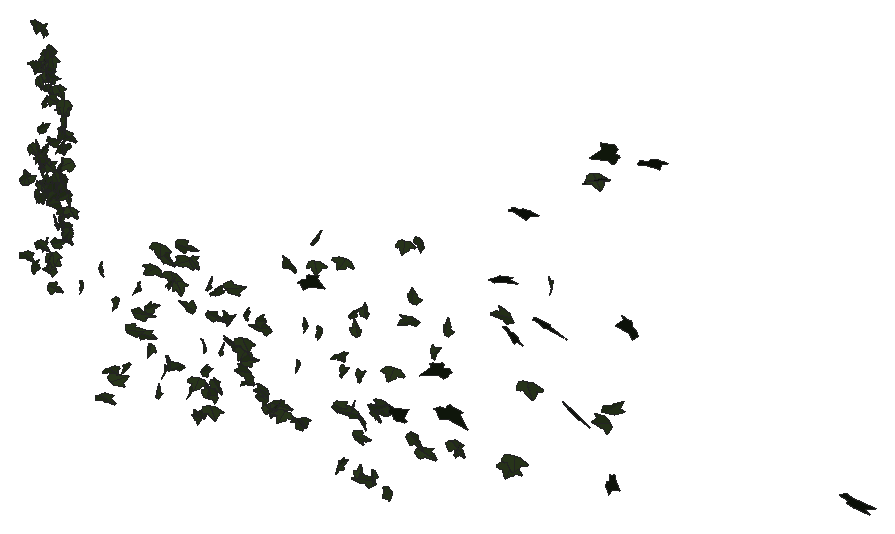
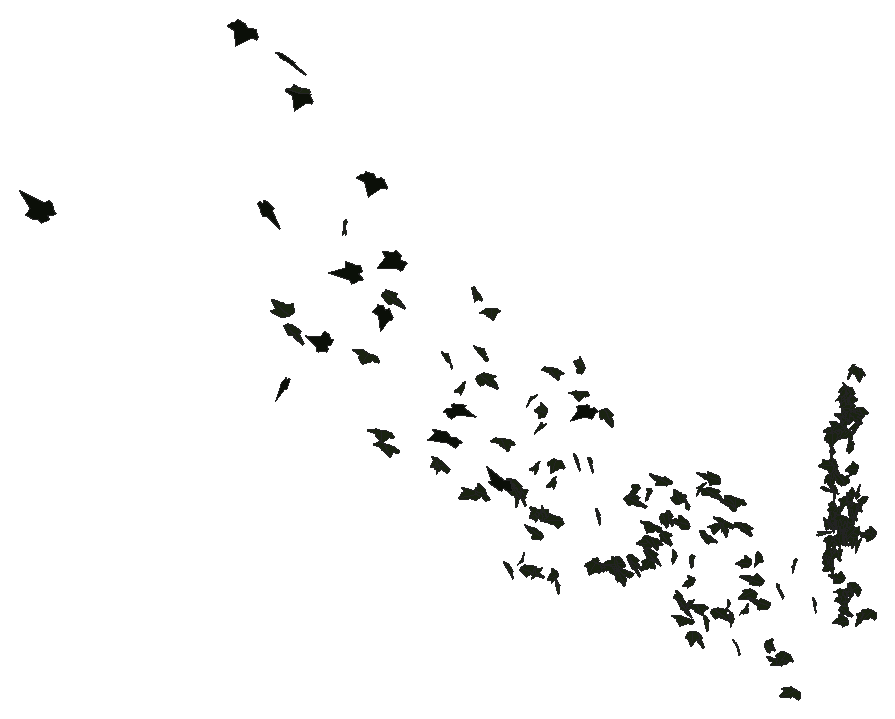
# SketchUp Ruby script. Lengths in millimetres.
U = 1.mm
M = Sketchup.active_model
def pt(a) = Geom::Point3d.new(a.map { |v| v * U })
def face(e, loops, mat)
  f = e.add_face(loops[0].map { |a| pt(a) })
  loops[1..].each { |l| e.add_face(l.map { |a| pt(a) }).erase! }
  f.material = f.back_material = mat if mat
  f
end
# faces: each face lists its corners as indices into pts; further lists are holes
def faces(e, pts, list, mat = nil) = list.each { |f| face(e, (f[0].is_a?(Array) ? f : [f]).map { |l| l.map { |i| pts[i] } }, mat) }
# xy, xz, yz: faces in a plane at the given z, y or x. An outline is a flat list of corners, or four numbers for a rectangle; further outlines are holes
def ring(l) = l.size == 4 ? [[l[0], l[1]], [l[2], l[1]], [l[2], l[3]], [l[0], l[3]]] : l.each_slice(2).to_a
def flat(e, list, mat, &to3) = list.each { |f| face(e, (f[0].is_a?(Array) ? f : [f]).map { |l| ring(l).map { |u, v| to3.(u, v) } }, mat) }
def xy(e, z, list, mat = nil) = flat(e, list, mat) { |x, y| [x, y, z] }
def xz(e, y, list, mat = nil) = flat(e, list, mat) { |x, z| [x, y, z] }
def yz(e, x, list, mat = nil) = flat(e, list, mat) { |y, z| [x, y, z] }
def lines(e, pts, list) = list.each { |a, b| e.add_line(pt(pts[a]), pt(pts[b])) }
# prism: a flat outline (further loops are holes) pulled along v
def prism(e, loops, v, mat = nil)
  f = face(e, loops, mat); d = Geom::Vector3d.new(v.map { |x| x * U })
  f.pushpull(f.normal.samedirection?(d) ? d.length : -d.length)
end
def box(e, o, s, mat = nil) = prism(e, [[o, [o[0] + s[0], o[1], o[2]], [o[0] + s[0], o[1] + s[1], o[2]], [o[0], o[1] + s[1], o[2]]]], [0, 0, s[2]], mat)
def at(x, y, z, deg = 0) = Geom::Transformation.translation(pt([x, y, z])) * Geom::Transformation.rotation(ORIGIN, Z_AXIS, deg.degrees)
def axes(o, x, y, z) = Geom::Transformation.new([*x, 0, *y, 0, *z, 0, *pt(o).to_a, 1])
def part(name) = M.definitions.add(name)
# library, detail: a bought-in or finely detailed component or shape, given as its bounding box
def library(name, o, s) = part(name).tap { |d| box(d.entities, o, s) }
def detail(e, o, s) = box(e.add_group.entities, o, s)
def put(e, d, t, mat = nil) = e.add_instance(d, t).tap { |i| i.material = mat if mat }
def group(e, t, mat = nil) = e.add_group.tap { |g| g.transformation = t; g.material = mat if mat }.entities
root = M.entities
M.materials.add("efeu1").color = [18, 25, 13]
M.materials.add("efeu2").color = [43, 57, 29]
c1 = part("ivyleaf_10")
p = [[0,12.8,-0.8],[-1.5,51.3,-10.9],[-4.9,51,-11.6],[-13.6,26.5,-7.3],[-13.2,15.9,-4.6],[-21.1,19.3,-7.2],
  [-29.5,16.3,-8.3],[-29.2,8.3,-6.2],[-19.7,-9.8,0.5],[-7.6,-13,4],[1,-12.2,5.8],[-0.4,51.1,-11.1],
  [-1.5,51.1,-10.9],[1,-12.4,5.9],[16.9,-12.4,3.5],[35.1,9.1,-5.1],[35,12.9,-6.1],[20.5,16.4,-4.9],
  [15.8,15,-3.8],[15.3,27.6,-7.1],[12.8,31.3,-7.8]]
faces(c1.entities,p,[[0,1,2,3,4,5,6,7,8,9,10],[11,12,0,13,14,15,16,17,18,19,20]],"efeu2")
c2 = part("ivyleaf_9")
p = [[39.1,54.8,31.7],[34.5,51.8,30.2],[-5.3,25.2,17.3],[-17.9,28.3,20.9],[-21.6,21.7,17],[-20.2,4.3,5.3],
  [-22.9,-0.3,2.5],[-17.1,-4,-0.6],[-2,-2.1,-1.2],[-0.7,-15.4,-10.1],[16.6,-22.3,-16.7],[21.1,-15.1,-12.5],
  [32.7,-10.7,-11],[46.1,-1.8,-6.6],[30.8,11.2,3.8]]
faces(c2.entities,p,[[0,1,2,3,4,5,6,7,8,9,10,11,12,13,14]],"efeu1")
put(root,c1,axes([1417.2,1060.7,237.2],[0.00481,0.00823,0.65497],[-0.143,0.65065,-0.00789],[-1.2384,-0.0751,0.00345]))
put(root,c1,axes([847.1,1071.3,767.4],[0.27579,-0.61594,-0.22684],[-0.01202,0.23671,-0.65255],[0.8007,0.21571,0.06834]))
put(root,c2,axes([2730.5,1072.8,870.6],[1.36099,-0.29359,0.30538],[0.54746,-0.10333,-0.77292],[0.59187,0.77069,0.0127]))
put(root,c1,axes([1434.3,1071.8,440],[0.24904,-0.04769,0.62357],[1.1423,0.18856,-0.11153],[-0.33439,0.60861,0.08342]))
put(root,c1,axes([1433.5,1072.7,105.2],[1.05934,0.28952,0.18915],[0.31871,0.08794,-0.62741],[-0.57587,0.58126,0.00071]))
put(root,c1,axes([1847.2,1066,846.2],[0.34798,-0.60012,0.45518],[-0.14943,0.45066,0.6257],[-1.42571,-0.19371,0.04552]))
put(root,c1,axes([1718.8,1076.8,188.1],[0.90095,0.37363,-0.23743],[-0.35141,-0.14928,-0.60307],[-0.76574,0.50812,-0.00259]))
put(root,c1,axes([843.6,1070.7,828.9],[0.01979,-0.64952,-0.24261],[0.13234,0.24206,-0.64081],[0.83547,-0.02296,0.10725]))
put(root,c1,axes([1582,1061.5,493.4],[-0.02885,0.10194,0.6291],[-0.48234,0.57642,-0.09951],[-1.11289,-0.25247,0.02682]))
put(root,c1,axes([832.4,1066.8,542.8],[-0.36855,0.38808,-0.44475],[-0.31395,0.36304,0.49158],[0.64808,0.39656,-0.01478]))
put(root,c1,axes([1339.1,1077,594.4],[0.92186,0.07712,-0.4767],[-0.89317,-0.08395,-0.49043],[-0.2166,0.6744,-0.00653]))
put(root,c1,axes([1194.9,1062.3,381.9],[-0.05109,-0.13598,0.63034],[0.0985,0.6284,0.13776],[-1.2233,0.05628,-0.01523]))
put(root,c2,axes([1823.8,1062.2,704.9],[0.06022,-0.12649,-0.76017],[-0.18241,0.75426,-0.12949],[1.45526,0.09978,0.01523]))
put(root,c1,axes([851.6,1074.5,982.4],[0.52934,0.52433,-0.07138],[-0.05892,-0.05268,-0.68056],[-0.64288,0.43655,0.00361]))
put(root,c1,axes([1649.9,1067.2,226.8],[0.5581,-0.38266,-0.5931],[-0.69671,0.46666,-0.48208],[1.14853,0.46902,-0.00423]))
put(root,c1,axes([1099.1,1084.1,135],[0.12569,-0.45119,0.46437],[0.08625,-0.46241,-0.45573],[1.22923,0.07858,-0.0155]))
put(root,c1,axes([1178.8,1066,283.4],[-0.45772,-0.26948,-0.52768],[0.68844,0.38427,-0.36111],[0.89313,-0.43431,0.00791]))
put(root,c1,axes([2627.1,1075.1,346.6],[1.37258,0.27698,0.03221],[0.05707,0.01177,-0.77256],[-0.52763,0.72182,0.00023]))
put(root,c1,axes([2388.3,1077,315],[0.93628,-0.01391,0.55242],[1.04983,-0.0318,-0.49203],[0.06279,0.73904,-0.01077]))
put(root,c1,axes([1559.3,1074.1,389.2],[1.13118,0.14862,0.25352],[0.45961,0.07893,-0.61243],[-0.31871,0.64133,0.01662]))
put(root,c1,axes([1452.1,1074.9,519.5],[-0.33025,-0.63394,0.08937],[0.05216,0.08516,0.65725],[-1.21733,0.17563,0.00391]))
put(root,c1,axes([744.3,1074.3,1085.4],[-0.66863,-0.33572,0.07291],[-0.0848,-0.02607,-0.64256],[0.41046,-0.55227,-0.01399]))
put(root,c1,axes([1631.8,1062.3,490.4],[0.03397,0.25278,0.58916],[-0.17207,0.58449,-0.24804],[-1.20793,-0.07615,0.0519]))
put(root,c1,axes([1057.8,1067.1,78.9],[0.73804,0.02328,-0.51446],[0.85489,0.29969,0.35215],[0.47937,-0.5703,0.16405]))
put(root,c1,axes([2047.3,1064.8,658.8],[0.1271,0.53267,-0.42449],[-0.00484,0.42672,0.53507],[1.29631,-0.05063,0.04362]))
put(root,c1,axes([777.1,1065.3,1221.3],[-0.2531,0.53421,0.39539],[-0.16532,0.3715,-0.57304],[-0.79379,-0.2477,-0.00672]))
put(root,c1,axes([1243.8,1079.5,576.9],[0.36883,-0.02855,0.63402],[1.17176,-0.15246,-0.19505],[0.2932,0.64521,-0.01804]))
put(root,c1,axes([1578,1069.6,287.9],[0.65752,-0.25995,-0.6108],[-0.89974,0.38703,-0.43212],[0.8869,0.58536,0.01446]))
put(root,c1,axes([867,1084.2,770.2],[-0.75924,0.29011,0.36104],[-0.51572,-0.6029,-0.24419],[0.23091,-0.39263,0.64174]))
put(root,c1,axes([2070.5,1080.7,99.9],[-0.04522,0.55589,-0.39749],[0.00246,-0.3977,-0.55625],[-1.30061,-0.02008,0.01277]))
put(root,c1,axes([1042.7,1070.5,111.8],[-0.69334,-0.43342,-0.3087],[0.41708,0.21872,-0.56569],[0.92285,-0.42447,0.02373]))
put(root,c1,axes([2787,1059.6,1017.5],[0.12788,-0.15203,-0.82381],[-0.14117,0.82213,-0.15777],[1.58809,0.08533,0.05231]))
put(root,c1,axes([2026.5,1061.5,432.2],[0.10352,0.0674,-0.67068],[0.2713,0.6565,0.07754],[1.25386,-0.14761,0.0386]))
put(root,c1,axes([1700.4,1072.7,218.8],[-0.00793,-0.63198,-0.20325],[-0.00251,0.20326,-0.63199],[1.26346,-0.00356,-0.00253]))
put(root,c1,axes([871.1,1081.8,609.4],[-0.33773,-0.62901,0.01414],[0.75646,-0.27537,-0.11044],[0.13021,-0.03172,0.6783]))
put(root,c1,axes([748.2,1075.3,1225.8],[-0.81266,0.06782,0.13447],[-0.17703,-0.12568,-0.65539],[-0.04921,-0.66783,0.137]))
put(root,c1,axes([757.4,1072.8,453.6],[-0.54125,-0.03239,-0.53298],[0.64951,0.02646,-0.44476],[0.0501,-0.69296,0.00793]))
put(root,c1,axes([804.2,1084.5,639.2],[-0.17556,-0.45275,0.43683],[-0.06899,-0.43699,-0.47154],[0.76443,-0.14341,0.05777]))
put(root,c1,axes([1422.6,1067.5,154.4],[0.03332,0.5523,-0.32851],[-0.01654,0.3288,0.55233],[1.22291,-0.0106,0.01642]))
put(root,c1,axes([2410.9,1063,298.1],[0.22768,-0.23907,0.6877],[-0.47086,0.6421,0.26625],[-1.3032,-0.27376,0.02394]))
put(root,c1,axes([1510.5,1070.8,560.1],[0.61861,0.02522,-0.59187],[1.09941,0.1362,0.32304],[0.24999,-0.66137,0.04396]))
put(root,c1,axes([1313.7,1074.2,643.3],[-0.05035,0.01832,-0.68042],[1.2934,-0.0376,-0.02743],[-0.07289,-0.6799,-0.01681]))
put(root,c1,axes([1255.7,1068.5,179.3],[0.17291,-0.50518,-0.45873],[-0.09673,0.45648,-0.51277],[1.2951,0.10154,0.02295]))
put(root,c1,axes([2019.2,1077.9,277.4],[-0.71041,0.48049,-0.3051],[0.32241,-0.25453,-0.60811],[-1.03416,-0.40942,0.02]))
put(root,c2,axes([2573.3,1062.9,969.9],[1.04965,0.38294,0.36968],[0.55991,0.22432,-0.67127],[-0.8442,0.62491,0.01443]))
put(root,c1,axes([751.8,1076.5,784.8],[-0.52623,0.5179,0.06245],[0.04431,-0.05102,0.67398],[0.63487,0.43284,0.00473]))
put(root,c1,axes([1005,1065.2,453],[-0.34031,0.34148,0.51919],[-0.46677,0.45762,-0.38545],[-1.08668,-0.3035,0.00297]))
put(root,c1,axes([782.1,1079.7,1124],[0.29169,-0.6235,0.08478],[0.04682,-0.07607,-0.66771],[0.76624,0.242,0.00853]))
put(root,c1,axes([1994.3,1081.5,282.4],[-0.1471,-0.06632,0.66836],[-1.06912,-0.36239,-0.10092],[0.70067,-0.56688,-0.01368]))
put(root,c1,axes([1945.7,1072.1,477.9],[-0.59228,-0.52985,-0.27677],[0.27258,0.23685,-0.61448],[1.10457,-0.34256,0.00323]))
put(root,c1,axes([1256.9,1080.8,218.7],[-0.20271,0.54055,-0.34534],[0.12751,-0.33878,-0.55094],[-1.21412,-0.12583,-0.0002]))
put(root,c1,axes([849.3,1080.7,924.5],[0.59209,-0.39807,0.16573],[0.16366,-0.09775,-0.62762],[0.49995,0.50343,0.00918]))
put(root,c2,axes([3096.9,1068.7,980.9],[0.16032,0.0511,-0.878],[-1.67294,0.03366,-0.08237],[0.05459,0.88139,0.05405]))
put(root,c1,axes([1842.6,1076,761.9],[0.85179,0.45412,0.03932],[0.05704,0.02566,-0.63759],[-0.86564,0.44855,-0.00332]))
put(root,c2,axes([3951.3,1082,659.3],[1.60991,0.03552,-0.51662],[0.97268,0.10211,0.84384],[0.15874,-0.98591,0.06879]))
put(root,c1,axes([1996.4,1066.6,636.9],[0.21824,-0.34911,0.56753],[-0.05846,0.5725,0.35837],[-1.26678,-0.08657,0.08124]))
put(root,c1,axes([796.2,1079.3,1153.7],[0.63727,-0.42194,-0.0248],[-0.02354,0.01557,-0.67148],[0.51511,0.5227,-0.00001]))
put(root,c1,axes([1645.9,1073.3,244.2],[0.60687,-0.23708,-0.51009],[-0.78048,0.30335,-0.39735],[0.73274,0.51947,-0.00077]))
put(root,c1,axes([808.5,1067,985],[0.13704,0.42379,0.47531],[0.04534,0.47747,-0.43449],[-0.77558,0.1028,0.05858]))
put(root,c1,axes([797.3,1068.9,746.8],[0.2059,0.51805,0.38799],[0.08407,0.3843,-0.5431],[-0.78514,0.17701,0.0436]))
put(root,c1,axes([1792.1,1069.5,173.4],[-0.30967,0.16443,-0.63572],[-0.83417,0.4605,0.23129],[0.93057,0.46751,-0.00423]))
put(root,c1,axes([847.3,1070.4,969.8],[0.33154,0.53,0.36014],[0.15557,0.33864,-0.59458],[-0.76612,0.29813,0.03512]))
put(root,c1,axes([772.1,1088.6,685.5],[0.09705,-0.33999,0.5387],[0.26814,-0.4949,-0.3448],[0.72944,0.22716,0.05507]))
put(root,c1,axes([778.6,1078.4,1115.6],[0.56949,0.46114,-0.07733],[-0.07821,-0.04513,-0.65604],[-0.56506,0.471,0.01286]))
put(root,c1,axes([769,1066,864.8],[0.07158,-0.20788,0.63337],[0.01131,0.63601,0.20788],[-0.81319,-0.00945,0.05865]))
put(root,c1,axes([804.5,1071.4,317],[0.18921,0.12201,0.62426],[0.59604,0.3886,-0.19733],[-0.49691,0.51258,0.00101]))
put(root,c1,axes([2603.5,1075.6,840.7],[-0.5503,0.06197,0.75697],[-1.44547,-0.02019,-0.28846],[-0.00607,-0.81006,0.0651]))
put(root,c1,axes([2268.8,1070.2,251.5],[0.60185,0.28971,0.5744],[0.725,0.43144,-0.42733],[-0.98665,0.49375,0.03637]))
put(root,c1,axes([1519,1069.3,368.9],[0.52313,-0.00481,-0.58183],[-0.67388,0.50924,-0.17148],[0.87874,0.39339,0.21487]))
put(root,c1,axes([768,1072.1,626.5],[0.07821,0.61309,0.20589],[-0.1975,0.21552,-0.59138],[-0.7639,0.00704,0.17398]))
put(root,c1,axes([1204.9,1079.2,519.3],[1.06621,0.0038,-0.30246],[-0.57529,0.03091,-0.55948],[0.0216,0.6359,0.029]))
put(root,c1,axes([805,1076.8,1116],[0.14795,0.66909,-0.01265],[-0.0001,-0.01284,-0.67999],[-0.81643,0.12125,-0.00221]))
put(root,c1,axes([2004.9,1083,206.1],[0.26605,-0.09929,-0.65288],[1.07345,-0.32916,0.17083],[-0.65373,-0.5809,0.0148]))
put(root,c1,axes([2145.6,1080.4,488.2],[1.19375,0.29443,-0.13824],[-0.23927,-0.05749,-0.6929],[-0.57093,0.63971,0.00135]))
put(root,c1,axes([797.1,1083.8,414.8],[-0.07628,0.54809,-0.35241],[-0.22222,-0.35461,-0.51921],[-0.76328,0.04847,0.18638]))
put(root,c1,axes([804.4,1077.4,426.5],[0.57735,0.47123,0.07495],[0.06615,0.05178,-0.66784],[-0.57836,0.47633,-0.00156]))
put(root,c1,axes([840.2,1075.1,570.4],[-0.1762,0.63364,0.06608],[-0.01472,0.06502,-0.64989],[-0.77709,-0.14491,-0.00268]))
put(root,c1,axes([1226.1,1080,604],[1.23606,0.10897,0.06347],[0.11855,0.0123,-0.65854],[-0.20868,0.65244,0.00181]))
put(root,c1,axes([1414.1,1066.8,320.7],[0.15197,-0.01841,-0.68233],[-0.34215,0.66217,-0.03891],[1.25323,0.18301,0.07212]))
put(root,c1,axes([794.2,1078.2,1138.9],[0.10726,0.65998,-0.05919],[-0.09481,-0.04903,-0.66209],[-0.80283,0.09396,0.07028]))
put(root,c1,axes([2216.6,1084.7,278],[0.60982,-0.11567,0.69432],[1.28068,-0.17348,-0.33944],[0.39303,0.74475,0.02877]))
put(root,c1,axes([1187.5,1085.5,232.7],[0.1469,0.49273,-0.40019],[-0.13805,-0.39365,-0.49867],[-1.20018,0.10559,0.00838]))
put(root,c1,axes([1499,1072,452.1],[0.44751,-0.34657,-0.49904],[-0.36102,0.46648,-0.41334],[1.09854,0.29449,0.06746]))
put(root,c1,axes([1952.5,1081.5,807.5],[1.19112,0.0799,-0.18006],[-0.33736,-0.03317,-0.63085],[-0.16354,0.65039,-0.01006]))
put(root,c1,axes([782.5,1076.5,1130.7],[-0.22263,0.65464,0.02724],[-0.00833,0.02637,-0.6796],[-0.79931,-0.18261,-0.0005]))
put(root,c1,axes([697.9,1067.8,658],[-0.01012,-0.19145,0.674],[0.17574,0.65918,0.18901],[-0.83655,0.14079,0.03156]))
put(root,c2,axes([2361.9,1078.8,426],[-0.26158,-0.26779,-0.74332],[1.07283,0.49543,-0.28271],[1.05363,-0.57094,0.10332]))
put(root,c1,axes([770.6,1084.2,757.6],[0.01788,-0.07944,0.63931],[0.76579,-0.14218,-0.03205],[0.17691,0.62347,0.07415]))
put(root,c1,axes([848.2,1079.4,962.2],[-0.53671,-0.49602,-0.01808],[0.0145,0.01362,-0.663],[0.60538,-0.44009,-0.00015]))
put(root,c1,axes([844.3,1078.5,588],[0.31856,-0.55773,-0.19964],[-0.10572,0.17987,-0.61582],[0.71493,0.27511,-0.00211]))
put(root,c1,axes([1385.5,1072.6,60.4],[0.42286,-0.28036,-0.54057],[-0.54013,0.46143,-0.35597],[1.02538,0.35869,0.03541]))
put(root,c1,axes([2053.9,1082.3,66.4],[0.40059,0.0558,-0.64674],[-1.23103,-0.03941,-0.21391],[-0.10437,0.67899,0.04074]))
put(root,c1,axes([748.5,1081.2,1078.2],[0.76991,-0.04681,-0.10964],[-0.13163,0.02705,-0.63253],[0.06188,0.63995,0.01871]))
put(root,c1,axes([1351.7,1076.4,135.9],[0.20544,-0.56389,-0.28607],[-0.12702,0.27842,-0.574],[1.19667,0.12636,-0.01182]))
put(root,c1,axes([790.3,1077.8,1144.4],[-0.5964,-0.41605,-0.19531],[0.22231,0.08632,-0.63997],[0.51477,-0.5193,0.0501]))
put(root,c1,axes([779.7,1080.3,1065.7],[-0.25011,0.60664,-0.15783],[0.07414,-0.14605,-0.64026],[-0.76114,-0.21357,-0.0105]))
put(root,c1,axes([1576.1,1072.5,255.4],[-0.43113,-0.3895,-0.44968],[0.41487,0.39336,-0.45054],[1.05349,-0.31431,-0.0066]))
put(root,c1,axes([804.5,1079.3,677.5],[-0.14822,-0.6408,-0.11356],[0.08909,0.10137,-0.65013],[0.78894,-0.13183,0.05208]))
put(root,c1,axes([1005.3,1075.3,-0.3],[-0.82155,-0.18607,-0.43952],[0.76529,0.17746,-0.47006],[0.48934,-0.58993,-0.00277]))
put(root,c1,axes([708.7,1079.7,656.3],[0.50001,0.50459,0.164],[-0.12594,-0.12743,0.65006],[0.63493,-0.42265,-0.0002]))
put(root,c1,axes([2605.4,1082.1,308.3],[1.45537,0.07383,-0.06299],[-0.11921,-0.00663,-0.76825],[-0.14108,0.76726,-0.00058]))
put(root,c1,axes([793.2,1077.3,668.9],[-0.29809,0.58998,0.13728],[-0.34918,0.01802,-0.58684],[-0.65131,-0.27968,0.25178]))
put(root,c1,axes([751.5,1076.9,1031.4],[0.07482,0.63722,0.08643],[0.02453,0.08488,-0.64006],[-0.78414,0.06345,-0.01178]))
put(root,c1,axes([1053.7,1084.1,350.3],[0.70295,-0.56109,0.06381],[0.06393,-0.05428,-0.67174],[1.07285,0.37087,-0.00178]))
put(root,c1,axes([842.7,1079.2,714.2],[-0.65882,0.33285,-0.11259],[0.11113,-0.06676,-0.63429],[-0.41402,-0.54757,0.0089]))
put(root,c1,axes([1861,1078.4,528.1],[0.50145,-0.57507,-0.26481],[-0.22302,0.23757,-0.63252],[1.18412,0.28827,-0.00699]))
put(root,c2,axes([2838.7,1089.9,588.8],[0.75934,-0.53124,0.52752],[0.58505,-0.42879,-0.66432],[1.2992,0.50359,-0.00916]))
put(root,c1,axes([1274.2,1081.8,496.8],[-0.00298,-0.66588,-0.03591],[0.00153,0.03591,-0.66588],[1.26914,-0.00161,0.00072]))
put(root,c1,axes([2218.5,1086.4,688.1],[-0.70556,-0.33491,0.50786],[-0.73442,-0.33031,-0.49951],[0.89507,-0.53503,-0.00953]))
put(root,c1,axes([1746.4,1075.3,725.3],[-0.94751,0.20256,0.52864],[-0.96058,0.16004,-0.53665],[-0.488,-0.70831,0.02992]))
put(root,c1,axes([2088.9,1082.5,324.9],[-1.14041,-0.22011,0.27285],[0.51729,0.04956,0.63688],[-0.42138,0.65654,0.0434]))
put(root,c1,axes([798.9,1082.7,643.7],[-0.46067,-0.51329,0.03968],[0.03209,-0.06838,-0.63424],[0.62726,-0.37347,0.06159]))
put(root,c1,axes([2111,1079.8,354.8],[0.97034,-0.29969,-0.37154],[-0.59586,0.20041,-0.59128],[0.68577,0.59818,0.01196]))
put(root,c1,axes([1557.7,1082.9,347.2],[1.231,-0.0717,-0.12679],[-0.23924,0.01675,-0.65076],[0.14003,0.6589,0.00275]))
put(root,c1,axes([817.4,1075.8,713.4],[0.02288,0.63747,0.18583],[-0.0493,0.18665,-0.63622],[-0.80858,0.00666,0.04405]))
put(root,c1,axes([2316.1,1067.4,615.7],[0.15722,-0.01528,-0.72796],[0.27359,0.71855,0.00123],[1.35848,-0.14294,0.084]))
put(root,c1,axes([1142.5,1075.9,339.1],[-0.2632,-0.088,0.63625],[0.95789,0.3895,0.16327],[-0.75947,0.52176,-0.01458]))
put(root,c1,axes([1573.1,1069.7,324.2],[-0.02251,-0.06652,0.67021],[0.27277,0.65471,0.06751],[-1.25245,0.14378,0.00266]))
put(root,c1,axes([1660.8,1076.5,190.1],[0.67026,0.40626,0.36962],[0.46815,0.27592,-0.53764],[-0.93462,0.42955,-0.00423]))
put(root,c1,axes([2007.8,1075,575.7],[0.13644,0.66212,-0.24659],[-0.05433,0.25037,0.66396],[1.3436,-0.05711,0.05189]))
put(root,c1,axes([1691.4,1073.1,210.8],[0.29163,0.09847,0.63212],[0.72876,0.50659,-0.17174],[-0.97537,0.40794,0.06068]))
put(root,c1,axes([850.2,1080.8,549.7],[-0.61058,-0.42141,-0.07898],[0.07259,0.05195,-0.65427],[0.51801,-0.504,-0.00141]))
put(root,c1,axes([1642.3,1082.1,461.5],[0.46409,0.02609,-0.59989],[-1.1344,0.08886,-0.23842],[0.13827,0.64144,0.05743]))
put(root,c1,axes([1354.8,1078.6,430.5],[0.20324,0.103,0.62596],[-1.20253,0.07391,0.09563],[-0.10773,-0.63069,0.11343]))
put(root,c1,axes([743.7,1074.6,621.3],[-0.23144,0.57444,0.29303],[-0.12131,0.27574,-0.60492],[-0.77733,-0.21406,0.00715]))
put(root,c1,axes([852.5,1086.2,655],[0.29449,0.35743,-0.47239],[-0.57717,-0.19067,-0.38601],[-0.43492,0.49504,0.1924]))
put(root,c1,axes([818.7,1085.7,609.7],[-0.25491,-0.06185,0.6089],[-0.67084,-0.26354,-0.21545],[0.32786,-0.58733,0.03256]))
put(root,c1,axes([2081.2,1078.5,325.2],[0.6642,-0.44864,-0.39026],[-0.3859,0.33561,-0.56713],[1.06387,0.40183,0.03794]))
put(root,c1,axes([1142.7,1073.6,431.7],[-0.04285,-0.46202,-0.52873],[0.11585,0.52573,-0.46198],[1.33131,-0.06062,0.02318]))
put(root,c1,axes([859.2,1092.8,526.3],[-0.1797,-0.41469,0.46308],[-0.0006,-0.47582,-0.42626],[0.75838,-0.09864,0.10939]))
put(root,c1,axes([2130.8,1080.8,52.3],[0.72171,-0.49957,-0.29594],[-0.31884,0.2443,-0.62706],[1.05809,0.41437,0.0129]))
put(root,c1,axes([1359.7,1075.9,604.3],[-0.13775,0.63015,0.26909],[-0.04384,0.26819,-0.63425],[-1.30333,-0.07562,-0.0071]))
put(root,c1,axes([1112.3,1079,271.1],[0.23642,0.04086,-0.62839],[1.17551,0.11687,0.1297],[0.23348,-0.6298,-0.0167]))
put(root,c1,axes([2248.2,1085.5,979.4],[0.95765,-0.47093,0.13603],[0.38839,0.02401,-0.67175],[0.84822,0.52069,0.15401]))
put(root,c1,axes([753.9,1081.5,649.1],[-0.44583,-0.21605,0.5068],[0.56478,0.20928,0.42302],[-0.36438,0.58871,0.03561]))
put(root,c2,axes([2144,1086.7,328.7],[-0.47437,0.09443,0.71655],[0.96819,-0.51549,0.24489],[0.97709,0.55664,0.10522]))
put(root,c1,axes([2087.7,1077.1,315.1],[-0.63725,0.53964,0.27175],[-0.33073,0.21156,-0.63421],[-1.10133,-0.37578,0.03321]))
put(root,c1,axes([803.9,1086.5,403.6],[0.65891,0.29952,-0.17926],[-0.17741,-0.10715,-0.61718],[-0.38714,0.55888,-0.02226]))
put(root,c1,axes([1807.8,1075.5,533.3],[0.27971,-0.37067,-0.54822],[-0.32723,0.5209,-0.3983],[1.21623,0.2254,0.01892]))
put(root,c1,axes([1439.5,1080.5,156.2],[0.75222,-0.35197,-0.48398],[-0.69605,0.31703,-0.52922],[0.90149,0.53847,-0.00477]))
put(root,c1,axes([1219.7,1079.2,75.9],[0.70585,-0.43016,0.34434],[-0.40746,0.26997,0.56784],[-0.96628,-0.42806,0.01209]))
put(root,c1,axes([837.3,1083.2,871.7],[0.52906,-0.42287,-0.2621],[-0.21104,0.19784,-0.6054],[0.56909,0.46649,0.01916]))
put(root,c1,axes([722.7,1077.6,780.1],[0.04263,0.61428,0.27477],[0.00199,0.27506,-0.61514],[-0.82098,0.03256,0.01278]))
put(root,c1,axes([840.2,1083.7,676.8],[-0.62402,0.0438,0.39046],[-0.47933,-0.06202,-0.50773],[0.00374,-0.6405,0.07586]))
put(root,c1,axes([755.3,1082.8,746.2],[-0.80685,-0.06659,-0.00009],[0.0001,0.00003,-0.6647],[0.08124,-0.66135,-0.00002]))
put(root,c2,axes([2653.5,1076.5,1234.3],[1.10725,0.45882,-0.17486],[-0.27014,-0.10238,-0.7409],[-0.8946,0.5988,0.0073]))
put(root,c1,axes([2226.4,1081.6,764.4],[1.11431,-0.32915,0.24817],[-0.41226,0.12111,0.67167],[-0.6675,-0.62428,-0.00055]))
put(root,c1,axes([1371.1,1087.4,177.2],[0.99137,0.35059,-0.16954],[-0.26735,-0.09492,-0.62789],[-0.69127,0.5395,-0.0003]))
put(root,c1,axes([695,1081.4,391.1],[-0.62062,-0.17584,-0.37285],[0.42901,0.12397,-0.53823],[0.26246,-0.61841,-0.00188]))
put(root,c1,axes([845,1083.2,599.3],[-0.56201,-0.39192,-0.22314],[0.22828,0.12414,-0.6043],[0.50062,-0.49658,0.02505]))
put(root,c1,axes([1504.5,1089,447.9],[-0.15893,-0.62761,0.08149],[-0.00874,-0.08159,-0.63311],[1.20446,-0.08341,0.00616]))
put(root,c1,axes([838.9,1083.9,872.8],[-0.72655,0.28618,0.04859],[-0.07814,-0.02137,-0.65906],[-0.34541,-0.59713,0.04688]))
put(root,c1,axes([766.1,1085.3,435.2],[0.28805,-0.6075,0.09977],[-0.0396,0.09443,0.65175],[-0.75003,-0.2383,0.0039]))
put(root,c1,axes([2942.5,1083,1450],[0.94017,0.60753,0.18061],[0.20057,0.14707,-0.78295],[-1.18947,0.505,0.01073]))
put(root,c1,axes([1264.8,1088.4,514],[1.19341,-0.04298,0.16909],[0.3216,-0.00736,-0.62851],[0.08262,0.64941,0.00407]))
put(root,c1,axes([774.7,1075.8,1079.9],[0.03056,-0.31048,0.60151],[0.06769,0.60084,0.30782],[-0.82306,0.03789,0.04765]))
put(root,c1,axes([830.9,1083.2,664],[0.23689,-0.58124,-0.23123],[0.11682,0.26688,-0.59044],[0.75417,0.14123,0.16409]))
put(root,c1,axes([797,1085.2,818.6],[-0.49015,-0.16736,0.49239],[0.55377,0.19083,0.43523],[-0.30966,0.60617,-0.00107]))
put(root,c2,axes([3163.2,1075,1586.2],[1.041,0.62526,0.04511],[0.05839,0.03309,-0.83074],[-1.19166,0.54783,-0.0013]))
put(root,c1,axes([734.9,1075,361.8],[-0.00446,0.3676,0.57838],[-0.2415,0.55317,-0.35283],[-0.80045,-0.16894,0.10323]))
put(root,c1,axes([916.8,1082.5,355.2],[0.38308,-0.51218,-0.35191],[-0.11856,0.35141,-0.5471],[1.17674,0.20214,0.05944]))
put(root,c1,axes([851.9,1090.8,653.5],[0.62442,-0.10442,0.37587],[0.44855,-0.07812,-0.52236],[0.15907,0.63018,-0.00247]))
put(root,c1,axes([1677.2,1091.3,185.5],[-0.16222,-0.70397,0.12732],[-0.03879,-0.12578,-0.70909],[1.36098,-0.08749,-0.00504]))
put(root,c1,axes([793.8,1089,636.3],[0.51488,-0.49123,0.03566],[0.14444,0.0556,-0.63528],[0.58326,0.41987,0.12584]))
put(root,c1,axes([842.2,1091.5,900.1],[-0.38487,0.49004,-0.26927],[0.00348,-0.30776,-0.56342],[-0.68215,-0.27805,0.14905]))
put(root,c1,axes([759.7,1081.5,662.7],[0.33578,0.48236,0.34661],[0.19096,0.30962,-0.55516],[-0.69904,0.31628,0.01484]))
put(root,c1,axes([792.6,1091.3,632.7],[-0.16213,-0.62239,0.09259],[0.01707,-0.09753,-0.63553],[0.76748,-0.12931,0.0337]))
put(root,c1,axes([793.1,1090.9,1034.6],[0.38674,-0.55651,0.01484],[0.01393,-0.01058,-0.64044],[0.67904,0.31717,0.00468]))
put(root,c1,axes([765.8,1085.6,717],[-0.50717,0.18699,-0.46288],[-0.5092,0.2003,0.45576],[0.33416,0.58903,-0.00804]))
put(root,c1,axes([747.8,1087.6,724.8],[-0.36852,0.56658,-0.10533],[0.05353,-0.09597,-0.64204],[-0.70103,-0.30517,0.00635]))
put(root,c1,axes([785,1085.6,1042.5],[-0.20732,-0.16801,0.60796],[0.67919,0.25603,0.22636],[-0.36174,0.57701,0.07658]))
put(root,c1,axes([1978.9,1082.2,284.5],[0.49834,-0.48451,0.38681],[-0.29189,0.35622,0.55002],[-1.14327,-0.30214,0.02818]))
put(root,c1,axes([3002.9,1084.4,644.7],[-0.6324,-0.69013,0.41546],[0.3327,0.37693,0.76594],[-1.49655,0.37542,-0.00528]))
put(root,c1,axes([1292.6,1086.1,490.4],[0.46026,0.59832,0.10775],[0.07492,0.10031,-0.64535],[-1.15462,0.24502,0.00108]))
put(root,c1,axes([854.1,1091.5,527.9],[-0.71347,0.21974,-0.13617],[0.05811,-0.23945,-0.59095],[-0.30998,-0.55065,0.20263]))
put(root,c1,axes([792.9,1082.7,1093.8],[0.0055,0.60743,0.24342],[-0.18526,0.23775,-0.59047],[-0.77656,-0.05242,0.14259]))
put(root,c2,axes([2611.8,1082.6,784.4],[1.10971,-0.05687,-0.5647],[-1.06404,0.08188,-0.58551],[0.18603,0.80757,0.0196]))
put(root,c1,axes([766.6,1081.5,777.9],[0.12981,-0.42627,0.46938],[-0.14913,0.45322,0.43931],[-0.75903,-0.16195,-0.00604]))
put(root,c1,axes([797.4,1088.2,689.9],[-0.66474,-0.22754,-0.27438],[0.35457,0.0066,-0.58261],[0.25178,-0.61002,0.09604]))
put(root,c1,axes([811.3,1082.4,468.3],[-0.18181,-0.1891,0.59768],[0.46446,0.46077,0.2407],[-0.6076,0.4088,0.00516]))
put(root,c1,axes([746.7,1083.8,751.7],[0.14869,0.62067,0.20119],[-0.13044,0.2209,-0.61671],[-0.78524,0.08083,0.14054]))
put(root,c1,axes([759.1,1090.7,1068.9],[0.4495,0.03784,-0.52875],[-0.6467,0.0313,-0.36714],[0.00503,0.6437,0.04893]))
put(root,c1,axes([846.9,1091,507.4],[-0.61235,0.06422,-0.3958],[0.45183,-0.16882,-0.49704],[-0.18751,-0.61651,0.09488]))
put(root,c1,axes([771.7,1090.2,1076.1],[-0.2337,0.60654,-0.11976],[-0.05604,-0.13899,-0.63047],[-0.75218,-0.17809,0.08418]))
put(root,c1,axes([1926.6,1084.1,286],[-0.33277,-0.11704,-0.63146],[1.11442,0.23973,-0.20657],[0.50199,-0.60979,0.03999]))
put(root,c1,axes([1427.3,1096.8,186.8],[0.58123,-0.10631,0.59024],[1.03378,-0.23178,-0.32279],[0.48391,0.62284,-0.01938]))
put(root,c1,axes([797.8,1089.9,369.8],[0.32056,-0.07589,-0.57907],[-0.69103,0.12164,-0.27295],[0.17365,0.62416,-0.01722]))
put(root,c1,axes([1946.2,1077.9,415.2],[0.01667,-0.10271,-0.66128],[0.30858,0.64196,-0.09756],[1.23569,-0.15893,0.03328]))
put(root,c1,axes([1411.9,1087.4,522.4],[0.63898,-0.55507,0.20984],[-0.16618,0.19227,0.64828],[-1.11709,-0.34611,0.02359]))
put(root,c1,axes([849.4,1090.2,862.6],[-0.383,-0.01895,-0.5643],[0.68518,-0.07697,-0.30986],[-0.07094,-0.64115,0.05388]))
put(root,c1,axes([2353.7,1087.8,696.6],[1.05083,-0.5034,0.20296],[-0.2835,0.13786,0.74718],[-0.99335,-0.57188,0.00146]))
put(root,c1,axes([778,1080.4,1042.4],[0.24778,0.25998,-0.56722],[0.4292,0.44494,0.3299],[0.6287,-0.40622,-0.00167]))
put(root,c2,axes([2324.3,1103,548.8],[-0.08117,-0.0166,-0.77044],[-0.13494,-0.76827,0.02048],[-1.46043,0.07191,0.04093]))
put(root,c1,axes([1778.3,1088.3,181.8],[-0.88394,-0.38016,-0.22724],[0.33419,0.14424,-0.6002],[0.77385,-0.49653,-0.00037]))
put(root,c1,axes([776.2,1091.7,1004.6],[-0.65273,0.05999,-0.33972],[0.39928,-0.10993,-0.53485],[-0.13306,-0.62416,0.06155]))
put(root,c1,axes([1768.9,1087.3,371.2],[0.35168,-0.5391,-0.35135],[-0.1917,0.33681,-0.56977],[1.20958,0.21012,0.01185]))
put(root,c1,axes([794.9,1091.3,628],[-0.34242,-0.55376,0.16901],[0.10039,0.14777,0.6208],[-0.69919,0.29241,0.00636]))
put(root,c1,axes([828.8,1089.7,713.5],[-0.781,0.0879,0.00655],[-0.0079,0.00098,-0.64617],[-0.10724,-0.6402,-0.00009]))
put(root,c1,axes([1941.4,1078.6,82],[0.10201,-0.08951,0.69254],[-0.26835,0.67889,0.09866],[-1.30164,-0.14698,0.03394]))
put(root,c1,axes([770.3,1079.9,952.4],[0.11149,-0.06144,0.63775],[-0.29145,0.59448,0.0915],[-0.72529,-0.24833,0.06127]))
put(root,c1,axes([845.6,1093.4,820.3],[-0.38057,-0.55563,0.04178],[-0.01556,-0.04075,-0.63715],[0.6796,-0.31208,0.00881]))
put(root,c1,axes([2012.1,1083.5,66.5],[0.17149,0.5689,-0.35279],[0.10832,0.34817,0.57599],[1.26941,-0.10657,-0.00149]))
put(root,c1,axes([2981.1,1086.9,595.3],[0.8857,-0.31699,-0.65978],[-0.95632,0.43017,-0.5611],[1.01301,0.68325,0.04716]))
put(root,c1,axes([815.4,1090.8,1015.1],[0.6262,0.2033,0.33282],[0.3601,0.15706,-0.55114],[-0.31098,0.59123,0.03197]))
put(root,c1,axes([1285.4,1099,194.6],[-0.57416,-0.34945,0.45715],[-0.57717,-0.3421,-0.46163],[0.93068,-0.42774,-0.00426]))
put(root,c2,axes([3007.3,1094.6,1553.2],[-1.47692,0.29218,0.09392],[-0.16773,0.03248,-0.8292],[-0.55951,-0.78101,0.00065]))
put(root,c1,axes([2669,1093.4,614],[1.44611,0.2131,0.24281],[0.44286,0.06947,-0.78914],[-0.42651,0.79465,0.00387]))
put(root,c1,axes([1390.2,1091.5,73.4],[-0.45686,-0.5896,-0.15276],[0.14697,0.13341,-0.63626],[1.14983,-0.25132,0.02063]))
put(root,c2,axes([3002.7,1082.3,396.6],[0.37303,-0.26161,-0.79321],[-0.91585,0.63057,-0.32688],[1.29928,0.5196,-0.00268]))
put(root,c2,axes([2939.2,1080.7,1438.2],[0.75391,0.68525,0.1331],[0.11868,0.11769,-0.79149],[-1.32323,0.40098,0.00485]))
put(root,c1,axes([1930,1087.8,70.4],[0.20722,-0.48751,-0.43349],[-0.20532,0.41998,-0.49941],[1.22449,0.15292,-0.01038]))
put(root,c1,axes([2179.5,1095.2,943.4],[0.79289,0.54406,-0.10376],[-0.17828,-0.05876,-0.68418],[-1.03893,0.4253,0.03821]))
put(root,c1,axes([1465.5,1083,317],[0.17894,-0.17676,0.63852],[-0.50855,0.58002,0.19991],[-1.15383,-0.28306,0.01091]))
